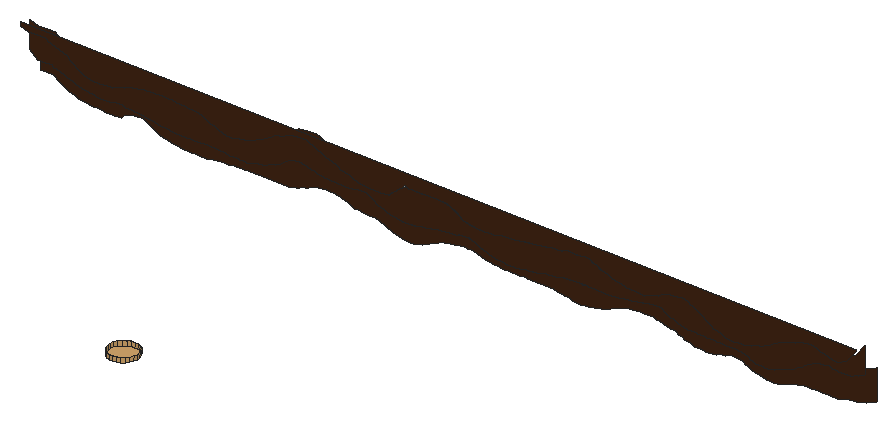
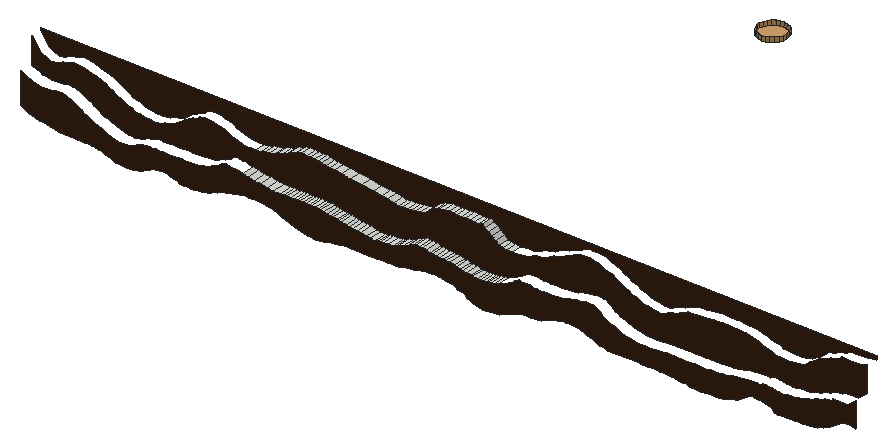
# SketchUp Ruby script. Lengths in inches.
U = 1.inch
M = Sketchup.active_model
def pt(a) = Geom::Point3d.new(a.map { |v| v * U })
def face(e, loops, mat)
  f = e.add_face(loops[0].map { |a| pt(a) })
  loops[1..].each { |l| e.add_face(l.map { |a| pt(a) }).erase! }
  f.material = f.back_material = mat if mat
  f
end
# faces: each face lists its corners as indices into pts; further lists are holes
def faces(e, pts, list, mat = nil) = list.each { |f| face(e, (f[0].is_a?(Array) ? f : [f]).map { |l| l.map { |i| pts[i] } }, mat) }
# xy, xz, yz: faces in a plane at the given z, y or x. An outline is a flat list of corners, or four numbers for a rectangle; further outlines are holes
def ring(l) = l.size == 4 ? [[l[0], l[1]], [l[2], l[1]], [l[2], l[3]], [l[0], l[3]]] : l.each_slice(2).to_a
def flat(e, list, mat, &to3) = list.each { |f| face(e, (f[0].is_a?(Array) ? f : [f]).map { |l| ring(l).map { |u, v| to3.(u, v) } }, mat) }
def xy(e, z, list, mat = nil) = flat(e, list, mat) { |x, y| [x, y, z] }
def xz(e, y, list, mat = nil) = flat(e, list, mat) { |x, z| [x, y, z] }
def yz(e, x, list, mat = nil) = flat(e, list, mat) { |y, z| [x, y, z] }
def lines(e, pts, list) = list.each { |a, b| e.add_line(pt(pts[a]), pt(pts[b])) }
# prism: a flat outline (further loops are holes) pulled along v
def prism(e, loops, v, mat = nil)
  f = face(e, loops, mat); d = Geom::Vector3d.new(v.map { |x| x * U })
  f.pushpull(f.normal.samedirection?(d) ? d.length : -d.length)
end
def box(e, o, s, mat = nil) = prism(e, [[o, [o[0] + s[0], o[1], o[2]], [o[0] + s[0], o[1] + s[1], o[2]], [o[0], o[1] + s[1], o[2]]]], [0, 0, s[2]], mat)
def at(x, y, z, deg = 0) = Geom::Transformation.translation(pt([x, y, z])) * Geom::Transformation.rotation(ORIGIN, Z_AXIS, deg.degrees)
def axes(o, x, y, z) = Geom::Transformation.new([*x, 0, *y, 0, *z, 0, *pt(o).to_a, 1])
def part(name) = M.definitions.add(name)
# library, detail: a bought-in or finely detailed component or shape, given as its bounding box
def library(name, o, s) = part(name).tap { |d| box(d.entities, o, s) }
def detail(e, o, s) = box(e.add_group.entities, o, s)
def put(e, d, t, mat = nil) = e.add_instance(d, t).tap { |i| i.material = mat if mat }
def group(e, t, mat = nil) = e.add_group.tap { |g| g.transformation = t; g.material = mat if mat }.entities
root = M.entities
M.materials.add("[Field Square Tile]").color = [211, 167, 108]
M.materials.add("[Wood Veneer 01]").color = [66, 38, 20]
xy(root,243.05,[[2115.79,563.18,2116.47,565.74]])
xy(root,243.07,[[2113.9375,563.18,2114.52,565.74]])
xy(root,243.09,[[2110.625,563.18,2111.15,565.74],[2111.15,563.18,2111.67,565.74],[2111.67,563.18,2112.33,565.74],[2112.33,563.18,2112.78,565.74]])
xy(root,249.21,[[2083.42,561.05,2084.31,563.18]])
xy(root,249.22,[[2085.03,561.05,2085.9375,563.18]])
xy(root,249.23,[[2086.58,561.05,2087.48,563.18]])
xy(root,250.6875,[[2081.97,492.77,2081.31,492.86,2080.69,493.11,2080.16,493.52,2079.75,494.05,2079.5,494.67,2079.41,495.33,2079.5,495.99,2079.75,496.61,2080.16,497.14,2080.69,497.55,2081.31,497.81,2081.97,497.89,2082.63,497.81,2083.25,497.55,2083.78,497.14,2084.19,496.61,2084.45,495.99,2084.53,495.33,2084.45,494.67,2084.19,494.05,2083.78,493.52,2083.25,493.11,2082.63,492.86]],"[Field Square Tile]")
xz(root,561.05,[[2141.84,244.87,2142.75,245.01,2143.6875,245.12,2144.45,245.25,2145.21,245.41,2145.84,245.78,2146.64,245.88,2147.35,246.16,2147.95,246.57,2148.74,246.9,2149.34,247.35,2150.01,247.62,2150.6,248.06,2151.36,248.32,2152.47,248.66,2153.25,248.79,2154.11,249.19,2154.78,249.32,2155.71,249.41,2156.56,249.48,2157.31,249.21,2157.95,248.96,2158.65,248.9,2159.45,248.42,2160.16,248.3,2160.87,248.22,2161.6875,248.56,2162.62,249.02,2164.35,251.16,2164.35,251.5,2010.34,251.5,2010.34,250.88,2011.93,250.53,2013.55,250.54,2015.01,250.55,2015.54,250.15,2016.15,249.97,2016.95,249.8,2017.62,249.41,2018.29,249.2,2019.06,249.01,2019.55,248.51,2020.18,248.07,2020.83,247.72,2021.47,247.25,2022.02,246.88,2022.74,246.73,2023.4,246.62,2024.14,246.54,2024.92,246.51,2025.7,246.58,2026.5,246.59,2027.3,246.69,2028.01,247.03,2028.7,247.2,2029.67,247.39,2030.3,247.78,2031.08,247.89,2032.08,248.18,2032.72,248.29,2033.61,248.35,2034.34,248.4,2035.33,248.4375,2035.99,248.46,2036.88,248.47,2037.62,248.48,2038.51,248.49,2039.24,248.39,2040.64,248.28,2041.67,248.15,2042.49,248.11,2043.29,248.08,2044.13,247.66,2044.76,247.46,2045.44,247.08,2046.125,246.94,2046.98,246.66,2047.59,246.35,2048.36,246.05,2049.26,246.13,2049.97,246.29,2050.77,246.41,2051.68,246.55,2052.41,246.92,2053.02,247.12,2053.7,247.31,2054.27,247.71,2055.2,248.03,2055.91,248.46,2056.69,248.82,2057.41,249.37,2058.2,249.5625,2059.1,249.9,2060.02,250.35,2060.68,250.49,2061.49,250.6,2062.51,250.58,2063.15,250.61,2063.77,250.32,2064.46,250.0625,2065.12,249.68,2065.88,249.46,2066.77,248.95,2067.99,248.69,2068.9,248.26,2069.5,247.9,2070.63,247.66,2071.21,247.53,2071.89,247.25,2072.7,246.95,2073.39,246.75,2074.18,246.66,2074.89,246.59,2075.78,246.55,2076.71,246.63,2077.45,246.74,2078.18,246.87,2078.79,247.42,2079.46,247.96,2080.03,248.44,2080.77,248.85,2081.24,249.34,2081.97,249.125,2082.74,249.17,2083.42,249.21,2084.31,249.21,2085.03,249.22,2085.9375,249.22,2086.58,249.23,2087.48,249.23,2088.22,249.24,2089.02,249.14,2089.65,248.82,2090.44,248.54,2091.14,248.04,2091.83,247.48,2092.72,247.29,2093.54,247.15,2094.27,247.05,2094.99,247,2095.9,246.96,2096.625,246.94,2097.54,247.04,2098.6,247.36,2099.78,247.43,2101.43,247.6,2103.41,247.98,2105.61,248.1875,2107.22,248.49,2108.47,248.62,2109.41,248.69,2110.09,248.75,2110.75,249.09,2111.45,249.18,2112.23,249.13,2112.93,249.17,2113.63,249.18,2114.53,249.29,2115.26,249.21,2115.87,248.8,2116.5625,248.73,2117.34,248.26,2118.04,248.02,2118.84,247.8125,2119.55,247.4,2120.46,247.27,2121.2,247.18,2122.125,246.91,2122.99,246.84,2123.94,246.79,2124.72,246.75,2125.47,246.83,2126.51,247.25,2127.38,247.55,2128.05,247.66,2128.68,248.16,2129.47,248.41,2130.17,248.52,2130.87,248.72,2131.57,248.8,2132.46,248.85,2133.29,248.6875,2133.83,248.26,2134.52,248.06,2135.41,247.55,2136.12,247.19,2136.93,246.63,2137.5625,246.13,2138.15,245.83,2138.83,245.67,2139.7,245.46,2140.41,245.0625,2141.125,244.95]],"[Wood Veneer 01]")
xz(root,563.18,[[2145.84,241.09,2146.41,241.14,2147.05,241.35,2147.64,241.46,2148.58,241.85,2149.58,242.23,2150.14,242.42,2150.86,242.61,2151.375,242.91,2151.75,243.14,2152.29,243.52,2152.77,243.71,2153.1,244.02,2153.54,244.21,2154.13,244.57,2154.6,244.76,2155.22,245.125,2155.72,245.32,2156.2,245.41,2156.75,245.48,2157.24,245.59,2157.77,245.55,2158.38,245.35,2158.87,245.31,2159.42,245.27,2159.98,245.24,2160.54,245.22,2161.1,245.34,2161.73,245.42,2162.3125,245.52,2162.69,245.76,2163.16,245.9,2164.35,246.43,2164.35,251.16,2162.62,249.02,2161.6875,248.56,2160.87,248.22,2160.16,248.3,2159.45,248.42,2158.65,248.9,2157.95,248.96,2157.31,249.21,2156.56,249.48,2155.71,249.41,2154.78,249.32,2154.11,249.19,2153.25,248.79,2152.47,248.66,2151.36,248.32,2150.6,248.06,2150.01,247.62,2149.34,247.35,2148.74,246.9,2147.95,246.57,2147.35,246.16,2146.64,245.88,2145.84,245.78,2145.21,245.41,2144.45,245.25,2143.6875,245.12,2142.75,245.01,2141.84,244.87,2141.125,244.95,2140.41,245.0625,2139.7,245.46,2138.83,245.67,2138.15,245.83,2137.5625,246.13,2136.93,246.63,2136.12,247.19,2135.41,247.55,2134.52,248.06,2133.83,248.26,2133.29,248.6875,2132.46,248.85,2131.57,248.8,2130.87,248.72,2130.17,248.52,2129.47,248.41,2128.68,248.16,2128.05,247.66,2127.38,247.55,2126.51,247.25,2125.47,246.83,2124.72,246.75,2123.94,246.79,2122.99,246.84,2122.125,246.91,2121.2,247.18,2120.46,247.27,2119.55,247.4,2118.84,247.8125,2118.04,248.02,2117.34,248.26,2116.5625,248.73,2115.87,248.8,2115.26,249.21,2114.53,249.29,2113.63,249.18,2112.93,249.17,2112.23,249.13,2111.45,249.18,2110.75,249.09,2110.09,248.75,2109.41,248.69,2108.47,248.62,2107.22,248.49,2105.61,248.1875,2103.41,247.98,2101.43,247.6,2099.78,247.43,2098.6,247.36,2097.54,247.04,2096.625,246.94,2095.9,246.96,2094.99,247,2094.27,247.05,2093.54,247.15,2092.72,247.29,2091.83,247.48,2091.14,248.04,2090.44,248.54,2089.65,248.82,2089.02,249.14,2088.22,249.24,2087.48,249.23,2086.58,249.23,2085.9375,249.22,2085.03,249.22,2084.31,249.21,2083.42,249.21,2082.74,249.17,2081.97,249.125,2081.24,249.34,2080.77,248.85,2080.03,248.44,2079.46,247.96,2078.79,247.42,2078.18,246.87,2077.45,246.74,2076.71,246.63,2075.78,246.55,2074.89,246.59,2074.18,246.66,2073.39,246.75,2072.7,246.95,2071.89,247.25,2071.21,247.53,2070.63,247.66,2069.5,247.9,2068.9,248.26,2067.99,248.69,2066.77,248.95,2065.88,249.46,2065.12,249.68,2064.46,250.0625,2063.77,250.32,2063.15,250.61,2062.51,250.58,2061.49,250.6,2060.68,250.49,2060.02,250.35,2059.1,249.9,2058.2,249.5625,2057.41,249.37,2056.69,248.82,2055.91,248.46,2055.2,248.03,2054.27,247.71,2053.7,247.31,2053.02,247.12,2052.41,246.92,2051.68,246.55,2050.77,246.41,2049.97,246.29,2049.26,246.13,2048.36,246.05,2047.59,246.35,2046.98,246.66,2046.125,246.94,2045.44,247.08,2044.76,247.46,2044.13,247.66,2043.29,248.08,2042.49,248.11,2041.67,248.15,2040.64,248.28,2039.24,248.39,2038.51,248.49,2037.62,248.48,2036.88,248.47,2035.99,248.46,2035.33,248.4375,2034.34,248.4,2033.61,248.35,2032.72,248.29,2032.08,248.18,2031.08,247.89,2030.3,247.78,2029.67,247.39,2028.7,247.2,2028.01,247.03,2027.3,246.69,2026.5,246.59,2025.7,246.58,2024.92,246.51,2024.14,246.54,2023.4,246.62,2022.74,246.73,2022.02,246.88,2021.47,247.25,2020.83,247.72,2020.18,248.07,2019.55,248.51,2019.06,249.01,2018.29,249.2,2017.62,249.41,2016.95,249.8,2016.15,249.97,2015.54,250.15,2015.01,250.55,2013.55,250.54,2011.93,250.53,2010.34,250.88,2010.34,246.2,2011.91,244.96,2013.3,244.9375,2014.55,244.92,2014.77,244.61,2015.33,244.54,2016.09,244.41,2016.76,244.11,2017.28,243.95,2017.94,243.79,2018.46,243.48,2019.1,243.3,2019.6875,243.14,2020.17,243.06,2020.89,242.85,2021.47,242.78,2022.28,242.73,2022.82,242.68,2023.49,242.51,2024.01,242.46,2024.55,242.58,2025.18,242.57,2025.81,242.81,2026.38,242.86,2026.94,242.89,2027.58,242.92,2028.01,242.625,2028.62,242.65,2029.17,242.62,2029.8,242.58,2030.36,242.57,2031,242.48,2031.66,242.38,2032.32,242.34,2032.99,242.24,2034.16,241.96,2034.93,241.89,2035.75,241.83,2036.35,241.78,2037.12,241.75,2037.57,241.74,2038.12,241.72,2039.38,241.7,2040.11,241.69,2040.78,241.68,2041.37,241.68,2041.86,241.67,2042.5625,241.74,2043.13,241.75,2045.13,241.75,2045.62,241.67,2046.15,241.66,2046.76,241.57,2047.3,241.53,2047.92,241.51,2048.47,241.49,2049.17,241.48,2049.83,241.47,2050.4,241.46,2051.11,241.6,2051.84,241.85,2052.51,241.91,2053.41,242.1,2054.18,242.46,2054.88,242.78,2055.65,242.97,2056.18,243.23,2056.58,243.48,2057.1,243.72,2057.4375,244.12,2057.91,244.39,2058.39,244.73,2058.875,244.87,2059.46,244.95,2060.14,245.01,2060.79,244.81,2061.36,244.7,2061.84,244.67,2062.45,244.55,2062.99,244.51,2063.45,244.25,2064.2,244.11,2064.76,244.04,2065.38,243.99,2066.1,243.95,2066.6,243.93,2067.29,243.91,2067.86,243.89,2068.56,243.88,2069.21,243.94,2069.85,243.95,2070.41,244.1,2071.04,244.13,2071.52,244.15,2072.04,244.17,2072.56,244.18,2073.16,243.8,2073.7,243.43,2074.31,243.09,2074.7,242.875,2075.2,242.68,2075.79,242.51,2076.3,242.21,2076.9,242.11,2077.58,241.96,2078.14,241.89,2078.6,241.85,2079.12,241.8125,2079.63,241.79,2080.21,241.78,2080.88,241.91,2081.35,241.93,2082.02,242.09,2082.79,242.2,2083.29,242.24,2083.9,242.42,2084.45,242.47,2085.2,242.71,2085.84,242.78,2086.32,242.82,2087.01,242.85,2087.71,242.87,2088.26,243.02,2088.88,243.05,2089.43,243.29,2090.11,243.35,2090.66,243.39,2091.26,243.42,2092.03,243.14,2092.6,242.9375,2093.15,242.65,2093.77,242.39,2094.53,242.14,2095.17,241.89,2095.66,241.78,2096.71,241.63,2097.48,241.56,2098.08,241.51,2098.53,241.48,2099.05,241.46,2099.92,241.51,2100.64,241.59,2101.58,241.82,2102.36,241.87,2103.125,241.98,2103.74,242.02,2104.39,242.19,2105.09,242.38,2105.58,242.4375,2106.1,242.48,2106.76,242.58,2107.29,242.61,2107.875,242.77,2108.33,242.95,2108.89,243.01,2109.4,243.05,2109.97,243.08,2110.625,243.09,2112.78,243.09,2113.35,243.08,2113.9375,243.07,2114.52,243.07,2115.18,243.0625,2115.79,243.05,2116.47,243.05,2117.74,243.1,2118.91,243.17,2120.05,243.4,2121.3125,243.52,2122.44,243.71,2123.34,243.99,2124.04,244.08,2124.74,244.21,2125.32,244.27,2125.86,244.3,2126.53,244.39,2127.125,244.19,2127.5,243.88,2127.98,243.59,2128.53,243.33,2129.08,243.22,2129.57,242.92,2130.05,242.75,2130.61,242.6,2131.17,242.52,2131.73,242.47,2132.3125,242.43,2132.89,242.4,2133.47,242.39,2134.05,242.37,2134.63,242.36,2135.22,242.35,2136.38,242.33,2136.96,242.33,2137.68,242.32,2138.15,242.3125,2138.79,242.3,2139.46,242.3,2139.91,242.29,2140.55,242.28,2141.0625,242.28,2141.69,242.2,2142.27,241.97,2142.84,241.84,2143.35,241.57,2143.77,241.33,2144.24,241.24,2144.77,241.17,2145.24,241.12]],"[Wood Veneer 01]")
xz(root,565.74,[[2079.2,236.98,2079.88,237.22,2080.73,237.43,2081.35,237.74,2082.05,238.02,2082.49,238.375,2083.05,238.51,2083.6875,238.76,2084.33,239.12,2084.91,239.22,2085.91,239.31,2086.72,239.54,2087.21,239.6,2087.83,239.65,2088.42,239.69,2088.98,239.7,2089.71,239.72,2090.32,239.56,2090.99,239.44,2091.84,239.16,2092.39,239.07,2093.16,238.93,2094.04,238.78,2094.52,238.73,2095.19,238.6875,2095.88,238.66,2096.55,238.65,2097.33,238.64,2097.95,238.63,2098.64,238.625,2099.5,238.625,2100.06,238.62,2104.95,238.62,2105.64,238.45,2106.4,238.25,2107.02,238.19,2107.79,238.15,2108.42,237.86,2109.19,237.79,2109.9,237.74,2110.77,237.87,2111.42,237.88,2112.54,238.14,2113.76,238.46,2114.51,238.72,2115.39,239.08,2116.18,239.375,2116.92,239.75,2117.57,239.97,2118.19,240.17,2118.87,240.27,2119.55,240.33,2120.24,240.37,2120.93,240.4,2121.625,240.41,2122.15,240.42,2122.73,240.43,2123.3,240.43,2123.95,240.27,2124.53,240.23,2125.18,239.96,2125.9375,239.8,2126.55,239.65,2127.3125,239.5,2127.9375,239.18,2128.62,239.01,2129.14,238.67,2129.71,238.56,2130.37,238.48,2130.9375,238.26,2131.51,238.19,2132.33,238.15,2132.86,238.11,2133.53,238.18,2134.21,238.18,2134.89,238.27,2135.41,238.55,2136.07,238.61,2136.66,238.66,2137.23,239.04,2137.97,239.125,2138.65,239.02,2139.34,238.96,2139.86,238.86,2140.36,238.57,2140.91,238.33,2141.62,238,2142.45,237.71,2142.99,237.59,2143.59,237.51,2144.18,237.45,2144.75,237.42,2145.48,237.4,2146.16,237.47,2146.76,237.5625,2147.45,237.84,2148.13,238.08,2148.82,238.33,2149.35,238.51,2149.92,238.6,2150.58,238.74,2151.16,238.8,2151.73,238.83,2152.47,238.86,2153.23,238.875,2153.77,238.88,2154.45,238.89,2155.13,238.89,2155.89,238.9,2157.28,238.9,2157.91,239.15,2158.68,239.28,2159.48,239.42,2160.2,239.49,2160.75,239.53,2161.4375,239.81,2161.96,239.96,2162.52,240.1,2164.35,240.89,2164.35,246.43,2163.16,245.9,2162.69,245.76,2162.3125,245.52,2161.73,245.42,2161.1,245.34,2160.54,245.22,2159.98,245.24,2159.42,245.27,2158.87,245.31,2158.38,245.35,2157.77,245.55,2157.24,245.59,2156.75,245.48,2156.2,245.41,2155.72,245.32,2155.22,245.125,2154.6,244.76,2154.13,244.57,2153.54,244.21,2153.1,244.02,2152.77,243.71,2152.29,243.52,2151.75,243.14,2151.375,242.91,2150.86,242.61,2150.14,242.42,2149.58,242.23,2148.58,241.85,2147.64,241.46,2147.05,241.35,2146.41,241.14,2145.84,241.09,2145.24,241.12,2144.77,241.17,2144.24,241.24,2143.77,241.33,2143.35,241.57,2142.84,241.84,2142.27,241.97,2141.69,242.2,2141.0625,242.28,2140.55,242.28,2139.91,242.29,2139.46,242.3,2138.79,242.3,2138.15,242.3125,2137.68,242.32,2136.96,242.33,2136.38,242.33,2135.22,242.35,2134.63,242.36,2134.05,242.37,2133.47,242.39,2132.89,242.4,2132.3125,242.43,2131.73,242.47,2131.17,242.52,2130.61,242.6,2130.05,242.75,2129.57,242.92,2129.08,243.22,2128.53,243.33,2127.98,243.59,2127.5,243.88,2127.125,244.19,2126.53,244.39,2125.86,244.3,2125.32,244.27,2124.74,244.21,2124.04,244.08,2123.34,243.99,2122.44,243.71,2121.3125,243.52,2120.05,243.4,2118.91,243.17,2117.74,243.1,2116.47,243.05,2115.79,243.05,2115.18,243.0625,2114.52,243.07,2113.9375,243.07,2113.35,243.08,2112.78,243.09,2110.625,243.09,2109.97,243.08,2109.4,243.05,2108.89,243.01,2108.33,242.95,2107.875,242.77,2107.29,242.61,2106.76,242.58,2106.1,242.48,2105.58,242.4375,2105.09,242.38,2104.39,242.19,2103.74,242.02,2103.125,241.98,2102.36,241.87,2101.58,241.82,2100.64,241.59,2099.92,241.51,2099.05,241.46,2098.53,241.48,2098.08,241.51,2097.48,241.56,2096.71,241.63,2095.66,241.78,2095.17,241.89,2094.53,242.14,2093.77,242.39,2093.15,242.65,2092.6,242.9375,2092.03,243.14,2091.26,243.42,2090.66,243.39,2090.11,243.35,2089.43,243.29,2088.88,243.05,2088.26,243.02,2087.71,242.87,2087.01,242.85,2086.32,242.82,2085.84,242.78,2085.2,242.71,2084.45,242.47,2083.9,242.42,2083.29,242.24,2082.79,242.2,2082.02,242.09,2081.35,241.93,2080.88,241.91,2080.21,241.78,2079.63,241.79,2079.12,241.8125,2078.6,241.85,2078.14,241.89,2077.58,241.96,2076.9,242.11,2076.3,242.21,2075.79,242.51,2075.2,242.68,2074.7,242.875,2074.31,243.09,2073.7,243.43,2073.16,243.8,2072.56,244.18,2072.04,244.17,2071.52,244.15,2071.04,244.13,2070.41,244.1,2069.85,243.95,2069.21,243.94,2068.56,243.88,2067.86,243.89,2067.29,243.91,2066.6,243.93,2066.1,243.95,2065.38,243.99,2064.76,244.04,2064.2,244.11,2063.45,244.25,2062.99,244.51,2062.45,244.55,2061.84,244.67,2061.36,244.7,2060.79,244.81,2060.14,245.01,2059.46,244.95,2058.875,244.87,2058.39,244.73,2057.91,244.39,2057.4375,244.12,2057.1,243.72,2056.58,243.48,2056.18,243.23,2055.65,242.97,2054.88,242.78,2054.18,242.46,2053.41,242.1,2052.51,241.91,2051.84,241.85,2051.11,241.6,2050.4,241.46,2049.83,241.47,2049.17,241.48,2048.47,241.49,2047.92,241.51,2047.3,241.53,2046.76,241.57,2046.15,241.66,2045.62,241.67,2045.13,241.75,2043.13,241.75,2042.5625,241.74,2041.86,241.67,2041.37,241.68,2040.78,241.68,2040.11,241.69,2039.38,241.7,2038.12,241.72,2037.57,241.74,2037.12,241.75,2036.35,241.78,2035.75,241.83,2034.93,241.89,2034.16,241.96,2032.99,242.24,2032.32,242.34,2031.66,242.38,2031,242.48,2030.36,242.57,2029.8,242.58,2029.17,242.62,2028.62,242.65,2028.01,242.625,2027.58,242.92,2026.94,242.89,2026.38,242.86,2025.81,242.81,2025.18,242.57,2024.55,242.58,2024.01,242.46,2023.49,242.51,2022.82,242.68,2022.28,242.73,2021.47,242.78,2020.89,242.85,2020.17,243.06,2019.6875,243.14,2019.1,243.3,2018.46,243.48,2017.94,243.79,2017.28,243.95,2016.76,244.11,2016.09,244.41,2015.33,244.54,2014.77,244.61,2014.55,244.92,2013.3,244.9375,2011.91,244.96,2010.34,246.2,2010.34,241.52,2011.55,241.69,2012.82,241.55,2013.84,240.85,2014.38,240.59,2014.98,240.2,2015.77,239.86,2016.22,239.64,2016.78,239.52,2017.29,239.19,2018.07,239.09,2018.76,239.03,2019.44,238.97,2020.14,238.94,2020.84,238.93,2021.53,238.92,2022.57,238.82,2023.08,238.8,2023.95,238.79,2024.69,238.77,2025.22,238.9375,2025.78,239.55,2026.36,239.69,2026.91,239.88,2027.64,239.99,2028.23,240.05,2028.89,240.09,2029.58,240.11,2030.28,239.71,2030.74,239.38,2031.32,239.11,2031.9,238.74,2032.55,238.43,2033.46,238.31,2033.93,238.21,2034.87,237.9,2035.53,237.82,2036.22,237.76,2036.93,237.71,2037.54,237.68,2038.14,237.67,2038.89,237.66,2039.58,237.65,2040.89,237.65,2041.56,237.89,2042.32,237.94,2042.9375,237.98,2043.79,238.1,2044.34,238.13,2045.1,238.15,2045.73,238.26,2046.48,238.28,2047.11,238.3,2047.96,238.32,2048.68,238.33,2049.91,238.33,2050.59,238.34,2056.16,238.34,2056.67,238.59,2057.49,238.72,2058.18,238.86,2058.69,239.18,2059.28,239.35,2059.84,239.52,2060.39,239.85,2061.03,240.03,2061.6875,240.12,2062.36,240.19,2063.125,240.23,2063.83,240.25,2064.45,240.27,2065.23,240.11,2065.86,239.92,2066.55,239.7,2067.08,239.53,2067.66,239.29,2068.32,239.04,2068.9,238.94,2069.47,238.875,2070.22,238.83,2070.98,238.8,2071.52,238.79,2072.19,238.78,2072.97,238.43,2073.75,238.28,2074.3125,237.96,2075.25,237.68,2075.92,237.33,2076.45,237.2,2077.14,237.11,2077.9,237.04,2078.59,237.01]],"[Wood Veneer 01]")
p = [[2097.48,563.18,241.56],[2097.48,565.74,241.56],[2098.08,565.74,241.51],[2098.08,563.18,241.51],[2098.53,565.74,241.48],[2098.53,563.18,241.48],
  [2099.05,565.74,241.46],[2099.05,563.18,241.46],[2099.92,565.74,241.51],[2099.92,563.18,241.51],[2100.64,565.74,241.59],[2100.64,563.18,241.59],
  [2095.66,563.18,241.78],[2095.66,565.74,241.78],[2096.71,565.74,241.63],[2096.71,563.18,241.63],[2101.58,565.74,241.82],[2101.58,563.18,241.82],
  [2078.14,563.18,241.89],[2078.14,565.74,241.89],[2078.6,565.74,241.85],[2078.6,563.18,241.85],[2079.12,565.74,241.8125],[2079.12,563.18,241.8125],
  [2079.63,565.74,241.79],[2079.63,563.18,241.79],[2080.21,565.74,241.78],[2080.21,563.18,241.78],[2080.88,565.74,241.91],[2080.88,563.18,241.91],
  [2095.17,563.18,241.89],[2095.17,565.74,241.89],[2102.36,565.74,241.87],[2102.36,563.18,241.87],[2077.58,563.18,241.96],[2077.58,565.74,241.96],
  [2081.35,565.74,241.93],[2081.35,563.18,241.93],[2082.02,565.74,242.09],[2082.02,563.18,242.09],[2094.53,563.18,242.14],[2094.53,565.74,242.14],
  [2103.125,565.74,241.98],[2103.125,563.18,241.98],[2076.9,563.18,242.11],[2076.9,565.74,242.11],[2103.74,565.74,242.02],[2103.74,563.18,242.02],
  [2104.39,565.74,242.19],[2104.39,563.18,242.19],[2076.3,563.18,242.21],[2076.3,565.74,242.21],[2082.79,565.74,242.2],[2082.79,563.18,242.2],
  [2093.77,563.18,242.39],[2093.77,565.74,242.39],[2083.29,565.74,242.24],[2083.29,563.18,242.24],[2083.9,565.74,242.42],[2083.9,563.18,242.42],
  [2105.09,565.74,242.38],[2105.09,563.18,242.38],[2084.45,565.74,242.47],[2084.45,563.18,242.47],[2093.15,563.18,242.65],[2093.15,565.74,242.65],
  [2105.58,565.74,242.4375],[2105.58,563.18,242.4375],[2106.1,565.74,242.48],[2106.1,563.18,242.48],[2085.2,565.74,242.71],[2085.2,563.18,242.71],
  [2106.76,565.74,242.58],[2106.76,563.18,242.58],[2092.6,563.18,242.9375],[2092.6,565.74,242.9375],[2107.29,565.74,242.61],[2107.29,563.18,242.61],
  [2107.875,565.74,242.77],[2107.875,563.18,242.77],[2085.84,565.74,242.78],[2085.84,563.18,242.78],[2086.32,565.74,242.82],[2086.32,563.18,242.82],
  [2087.01,565.74,242.85],[2087.01,563.18,242.85],[2108.33,565.74,242.95],[2108.33,563.18,242.95],[2087.71,565.74,242.87],[2087.71,563.18,242.87],
  [2088.26,565.74,243.02],[2088.26,563.18,243.02],[2092.03,563.18,243.14],[2092.03,565.74,243.14],[2088.88,565.74,243.05],[2088.88,563.18,243.05],
  [2108.89,565.74,243.01],[2108.89,563.18,243.01],[2109.4,565.74,243.05],[2109.4,563.18,243.05],[2109.97,565.74,243.08],[2109.97,563.18,243.08],
  [2116.47,563.18,243.05],[2116.47,565.74,243.05],[2117.74,565.74,243.1],[2117.74,563.18,243.1],[2089.43,565.74,243.29],[2089.43,563.18,243.29],
  [2091.26,563.18,243.42],[2091.26,565.74,243.42],[2110.625,565.74,243.09],[2110.625,563.18,243.09],[2112.78,563.18,243.09],[2112.78,565.74,243.09],
  [2113.35,565.74,243.08],[2113.35,563.18,243.08],[2113.9375,565.74,243.07],[2113.9375,563.18,243.07],[2114.52,563.18,243.07],[2114.52,565.74,243.07],
  [2115.18,565.74,243.0625],[2115.18,563.18,243.0625],[2115.79,565.74,243.05],[2115.79,563.18,243.05],[2118.91,565.74,243.17],[2118.91,563.18,243.17],
  [2120.05,565.74,243.4],[2120.05,563.18,243.4],[2090.11,565.74,243.35],[2090.11,563.18,243.35],[2090.66,565.74,243.39],[2090.66,563.18,243.39],
  [2121.3125,565.74,243.52],[2121.3125,563.18,243.52],[2122.44,565.74,243.71],[2122.44,563.18,243.71],[2123.34,565.74,243.99],[2123.34,563.18,243.99],
  [2075.78,561.05,246.55],[2075.78,563.18,246.55],[2076.71,563.18,246.63],[2076.71,561.05,246.63],[2077.45,563.18,246.74],[2077.45,561.05,246.74],
  [2078.18,563.18,246.87],[2078.18,561.05,246.87],[2122.125,561.05,246.91],[2122.125,563.18,246.91],[2122.99,563.18,246.84],[2122.99,561.05,246.84],
  [2078.79,563.18,247.42],[2078.79,561.05,247.42],[2095.9,561.05,246.96],[2095.9,563.18,246.96],[2096.625,563.18,246.94],[2096.625,561.05,246.94],
  [2097.54,563.18,247.04],[2097.54,561.05,247.04],[2121.2,561.05,247.18],[2121.2,563.18,247.18],[2093.54,561.05,247.15],[2093.54,563.18,247.15],
  [2094.27,563.18,247.05],[2094.27,561.05,247.05],[2094.99,563.18,247],[2094.99,561.05,247],[2098.6,563.18,247.36],[2098.6,561.05,247.36],
  [2092.72,561.05,247.29],[2092.72,563.18,247.29],[2120.46,561.05,247.27],[2120.46,563.18,247.27],[2091.83,561.05,247.48],[2091.83,563.18,247.48],
  [2119.55,561.05,247.4],[2119.55,563.18,247.4],[2079.46,563.18,247.96],[2079.46,561.05,247.96],[2099.78,563.18,247.43],[2099.78,561.05,247.43],
  [2101.43,563.18,247.6],[2101.43,561.05,247.6],[2118.84,561.05,247.8125],[2118.84,563.18,247.8125],[2091.14,561.05,248.04],[2091.14,563.18,248.04],
  [2103.41,563.18,247.98],[2103.41,561.05,247.98],[2118.04,561.05,248.02],[2118.04,563.18,248.02],[2080.03,563.18,248.44],[2080.03,561.05,248.44],
  [2090.44,561.05,248.54],[2090.44,563.18,248.54],[2105.61,563.18,248.1875],[2105.61,561.05,248.1875],[2117.34,561.05,248.26],[2117.34,563.18,248.26],
  [2107.22,563.18,248.49],[2107.22,561.05,248.49],[2116.5625,561.05,248.73],[2116.5625,563.18,248.73],[2080.77,563.18,248.85],[2080.77,561.05,248.85],
  [2089.65,561.05,248.82],[2089.65,563.18,248.82],[2108.47,563.18,248.62],[2108.47,561.05,248.62],[2109.41,563.18,248.69],[2109.41,561.05,248.69],
  [2110.09,563.18,248.75],[2110.09,561.05,248.75],[2115.87,561.05,248.8],[2115.87,563.18,248.8],[2089.02,561.05,249.14],[2089.02,563.18,249.14],
  [2110.75,563.18,249.09],[2110.75,561.05,249.09],[2115.26,561.05,249.21],[2115.26,563.18,249.21],[2081.24,563.18,249.34],[2081.24,561.05,249.34],
  [2081.97,563.18,249.125],[2081.97,561.05,249.125],[2082.74,563.18,249.17],[2082.74,561.05,249.17],[2088.22,561.05,249.24],[2088.22,563.18,249.24],
  [2111.45,563.18,249.18],[2111.45,561.05,249.18],[2112.23,563.18,249.13],[2112.23,561.05,249.13],[2112.93,563.18,249.17],[2112.93,561.05,249.17],
  [2083.42,563.18,249.21],[2083.42,561.05,249.21],[2084.31,561.05,249.21],[2084.31,563.18,249.21],[2085.03,563.18,249.22],[2085.03,561.05,249.22],
  [2085.9375,561.05,249.22],[2085.9375,563.18,249.22],[2086.58,563.18,249.23],[2086.58,561.05,249.23],[2087.48,561.05,249.23],[2087.48,563.18,249.23],
  [2113.63,563.18,249.18],[2113.63,561.05,249.18],[2114.53,563.18,249.29],[2114.53,561.05,249.29],[2081.97,492.77,251.5],[2081.31,492.86,251.5],
  [2081.31,492.86,250.6875],[2081.97,492.77,250.6875],[2082.63,492.86,251.5],[2082.63,492.86,250.6875],[2080.69,493.11,251.5],[2080.69,493.11,250.6875],
  [2083.25,493.11,251.5],[2083.25,493.11,250.6875],[2080.16,493.52,251.5],[2080.16,493.52,250.6875],[2083.78,493.52,251.5],[2083.78,493.52,250.6875],
  [2079.75,494.05,251.5],[2079.75,494.05,250.6875],[2084.19,494.05,251.5],[2084.19,494.05,250.6875],[2079.5,494.67,251.5],[2079.5,494.67,250.6875],
  [2084.45,494.67,251.5],[2084.45,494.67,250.6875],[2079.41,495.33,251.5],[2079.41,495.33,250.6875],[2084.53,495.33,251.5],[2084.53,495.33,250.6875],
  [2079.5,495.99,251.5],[2079.5,495.99,250.6875],[2084.45,495.99,251.5],[2084.45,495.99,250.6875],[2079.75,496.61,251.5],[2079.75,496.61,250.6875],
  [2084.19,496.61,251.5],[2084.19,496.61,250.6875],[2080.16,497.14,251.5],[2080.16,497.14,250.6875],[2083.78,497.14,251.5],[2083.78,497.14,250.6875],
  [2080.69,497.55,251.5],[2080.69,497.55,250.6875],[2083.25,497.55,251.5],[2083.25,497.55,250.6875],[2081.31,497.81,251.5],[2081.31,497.81,250.6875],
  [2082.63,497.81,251.5],[2082.63,497.81,250.6875],[2081.97,497.89,251.5],[2081.97,497.89,250.6875]]
faces(root,p,[[0,1,2,3],[3,2,4,5],[5,4,6,7],[7,6,8,9],[9,8,10,11],[12,13,14,15],[15,14,1,0],[11,10,16,17],
  [18,19,20,21],[21,20,22,23],[23,22,24,25],[25,24,26,27],[27,26,28,29],[30,31,13,12],[17,16,32,33],[34,35,19,18],
  [29,28,36,37],[37,36,38,39],[40,41,31,30],[33,32,42,43],[44,45,35,34],[43,42,46,47],[47,46,48,49],[50,51,45,44],
  [39,38,52,53],[54,55,41,40],[53,52,56,57],[57,56,58,59],[49,48,60,61],[59,58,62,63],[64,65,55,54],[61,60,66,67],
  [67,66,68,69],[63,62,70,71],[69,68,72,73],[74,75,65,64],[73,72,76,77],[77,76,78,79],[71,70,80,81],[81,80,82,83],
  [83,82,84,85],[79,78,86,87],[85,84,88,89],[89,88,90,91],[92,93,75,74],[91,90,94,95],[87,86,96,97],[97,96,98,99],
  [99,98,100,101],[102,103,104,105],[95,94,106,107],[108,109,93,92],[101,100,110,111],[112,113,114,115],[115,114,116,117],[118,119,120,121],
  [121,120,122,123],[105,104,124,125],[125,124,126,127],[107,106,128,129],[129,128,130,131],[131,130,109,108],[127,126,132,133],[133,132,134,135],
  [135,134,136,137],[138,139,140,141],[141,140,142,143],[143,142,144,145],[146,147,148,149],[145,144,150,151],[152,153,154,155],[155,154,156,157],
  [158,159,147,146],[160,161,162,163],[163,162,164,165],[165,164,153,152],[157,156,166,167],[168,169,161,160],[170,171,159,158],[172,173,169,168],
  [174,175,171,170],[151,150,176,177],[167,166,178,179],[179,178,180,181],[182,183,175,174],[184,185,173,172],[181,180,186,187],[188,189,183,182],
  [177,176,190,191],[192,193,185,184],[187,186,194,195],[196,197,189,188],[195,194,198,199],[200,201,197,196],[191,190,202,203],[204,205,193,192],
  [199,198,206,207],[207,206,208,209],[209,208,210,211],[212,213,201,200],[214,215,205,204],[211,210,216,217],[218,219,213,212],[203,202,220,221],
  [221,220,222,223],[223,222,224,225],[226,227,215,214],[217,216,228,229],[229,228,230,231],[231,230,232,233],[225,224,234,235],[236,237,238,239],
  [240,241,242,243],[244,245,227,226],[233,232,246,247],[247,246,248,249],[249,248,219,218]])
faces(root,p,[[250,251,252,253],[254,250,253,255],[251,256,257,252],[258,254,255,259],[256,260,261,257],[262,258,259,263],[260,264,265,261],[266,262,263,267],
  [264,268,269,265],[270,266,267,271],[268,272,273,269],[274,270,271,275],[272,276,277,273],[278,274,275,279],[276,280,281,277],[282,278,279,283],
  [280,284,285,281],[286,282,283,287],[284,288,289,285],[290,286,287,291],[288,292,293,289],[294,290,291,295],[292,296,297,293],[296,294,295,297]],"[Field Square Tile]")
